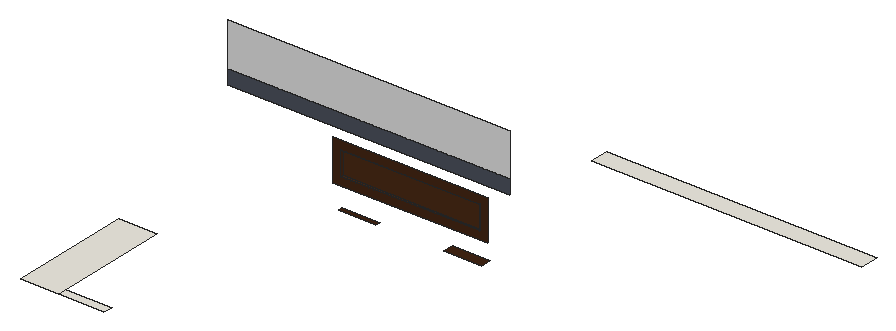
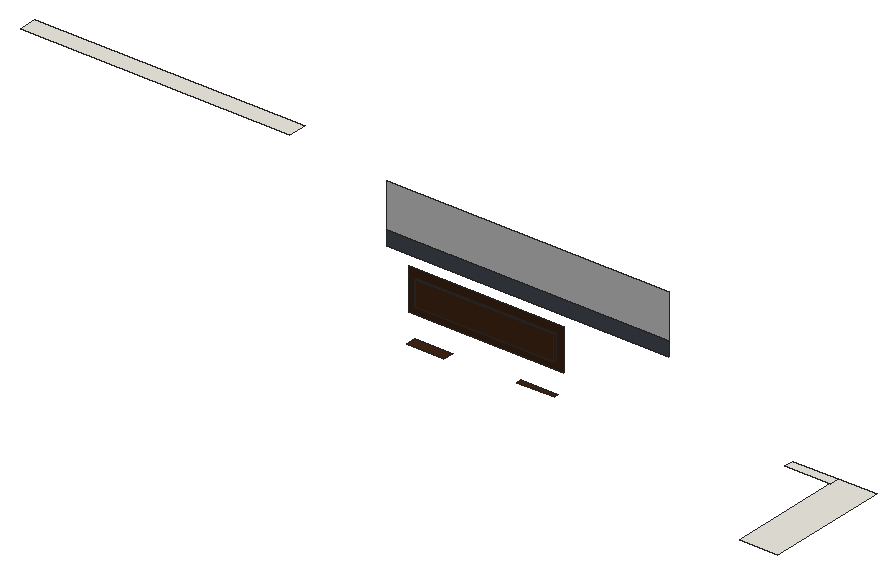
# SketchUp Ruby script. Lengths in inches.
U = 1.inch
M = Sketchup.active_model
def pt(a) = Geom::Point3d.new(a.map { |v| v * U })
def face(e, loops, mat)
  f = e.add_face(loops[0].map { |a| pt(a) })
  loops[1..].each { |l| e.add_face(l.map { |a| pt(a) }).erase! }
  f.material = f.back_material = mat if mat
  f
end
# faces: each face lists its corners as indices into pts; further lists are holes
def faces(e, pts, list, mat = nil) = list.each { |f| face(e, (f[0].is_a?(Array) ? f : [f]).map { |l| l.map { |i| pts[i] } }, mat) }
# xy, xz, yz: faces in a plane at the given z, y or x. An outline is a flat list of corners, or four numbers for a rectangle; further outlines are holes
def ring(l) = l.size == 4 ? [[l[0], l[1]], [l[2], l[1]], [l[2], l[3]], [l[0], l[3]]] : l.each_slice(2).to_a
def flat(e, list, mat, &to3) = list.each { |f| face(e, (f[0].is_a?(Array) ? f : [f]).map { |l| ring(l).map { |u, v| to3.(u, v) } }, mat) }
def xy(e, z, list, mat = nil) = flat(e, list, mat) { |x, y| [x, y, z] }
def xz(e, y, list, mat = nil) = flat(e, list, mat) { |x, z| [x, y, z] }
def yz(e, x, list, mat = nil) = flat(e, list, mat) { |y, z| [x, y, z] }
def lines(e, pts, list) = list.each { |a, b| e.add_line(pt(pts[a]), pt(pts[b])) }
# prism: a flat outline (further loops are holes) pulled along v
def prism(e, loops, v, mat = nil)
  f = face(e, loops, mat); d = Geom::Vector3d.new(v.map { |x| x * U })
  f.pushpull(f.normal.samedirection?(d) ? d.length : -d.length)
end
def box(e, o, s, mat = nil) = prism(e, [[o, [o[0] + s[0], o[1], o[2]], [o[0] + s[0], o[1] + s[1], o[2]], [o[0], o[1] + s[1], o[2]]]], [0, 0, s[2]], mat)
def at(x, y, z, deg = 0) = Geom::Transformation.translation(pt([x, y, z])) * Geom::Transformation.rotation(ORIGIN, Z_AXIS, deg.degrees)
def axes(o, x, y, z) = Geom::Transformation.new([*x, 0, *y, 0, *z, 0, *pt(o).to_a, 1])
def part(name) = M.definitions.add(name)
# library, detail: a bought-in or finely detailed component or shape, given as its bounding box
def library(name, o, s) = part(name).tap { |d| box(d.entities, o, s) }
def detail(e, o, s) = box(e.add_group.entities, o, s)
def put(e, d, t, mat = nil) = e.add_instance(d, t).tap { |i| i.material = mat if mat }
def group(e, t, mat = nil) = e.add_group.tap { |g| g.transformation = t; g.material = mat if mat }.entities
root = M.entities
M.materials.add("[Formica Laminate Dark]").color = [74, 78, 89]
M.materials.add("[Mirror 01]").color = [216, 216, 216]
M.materials.add("[Tile Limestone Large]").color = [237, 234, 224]
M.materials.add("[Wood Veneer 01]").color = [66, 38, 20]
M.materials.add("[Wood Veneer 01]1").color = [71, 41, 22]
xy(root,155.84,[[46.1875,137.79,76.4,233.86],[76.4,137.79,111.84,144.7]],"[Tile Limestone Large]")
xy(root,214.82,[[209.83,244.48,239.03,247.79],[292.21,244.48,321.41,252.61]],"[Wood Veneer 01]")
xy(root,238.6875,[[211.42,244.48,319.92,246.61]],"[Wood Veneer 01]1")
xy(root,257.68,[[211.42,244.48,319.92,246.61]],"[Wood Veneer 01]1")
xy(root,326.11,[[416.36,233.86,627.05,248.23]],"[Tile Limestone Large]")
xz(root,244.48,[[123.4,272.12,343.83,283.33]],"[Formica Laminate Dark]")
xz(root,244.48,[[123.4,283.33,343.83,317.47]],"[Mirror 01]")
xz(root,244.48,[[[205.03,232.3,326.31,264.07],[211.42,238.6875,319.92,257.68]]],"[Wood Veneer 01]")
xz(root,246.61,[[211.42,238.6875,319.92,257.68]],"[Wood Veneer 01]1")
yz(root,211.42,[[244.48,238.6875,246.61,257.68]],"[Wood Veneer 01]1")
yz(root,319.92,[[244.48,238.6875,246.61,257.68]],"[Wood Veneer 01]1")
